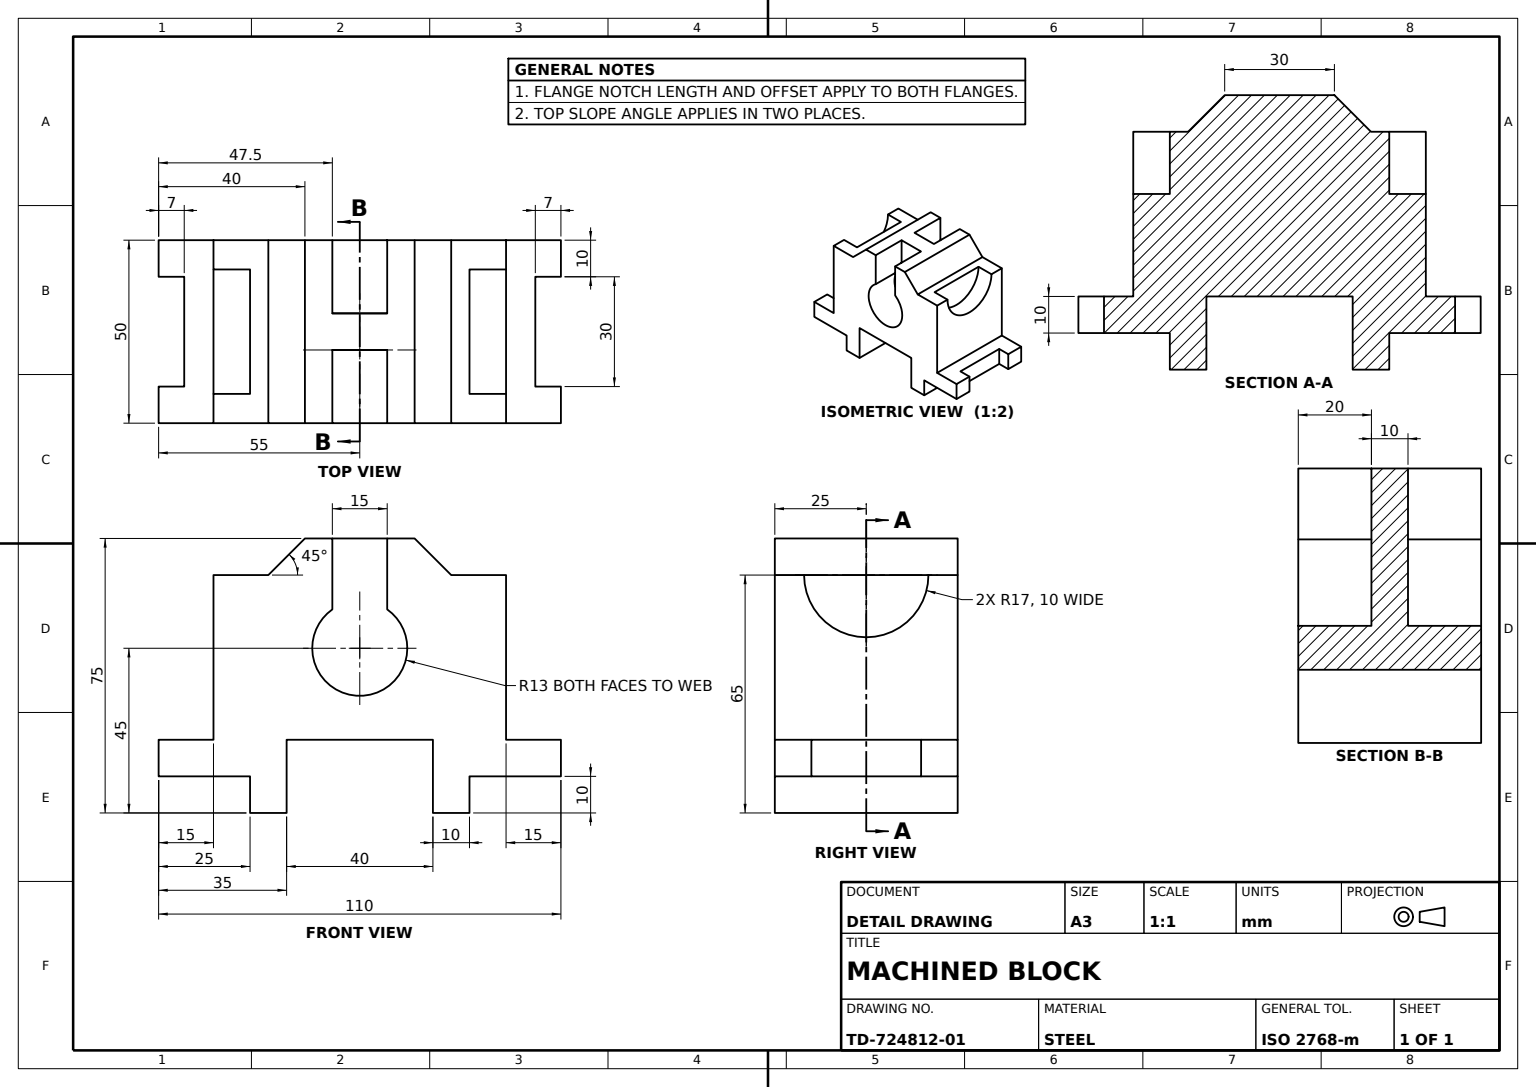
ISO-10303-21;
HEADER;
FILE_DESCRIPTION((''),'2;1');
FILE_NAME('','',(''),(''),'','','');
FILE_SCHEMA(('AUTOMOTIVE_DESIGN'));
ENDSEC;
DATA;
#1=APPLICATION_CONTEXT('');
#2=PRODUCT_CONTEXT('',#1,'mechanical');
#3=PRODUCT('','','',(#2));
#4=PRODUCT_DEFINITION_FORMATION('','',#3);
#5=PRODUCT_DEFINITION_CONTEXT('',#1,'design');
#6=PRODUCT_DEFINITION('','',#4,#5);
#7=PRODUCT_DEFINITION_SHAPE('','',#6);
#8=(LENGTH_UNIT()NAMED_UNIT(*)SI_UNIT(.MILLI.,.METRE.));
#9=(NAMED_UNIT(*)PLANE_ANGLE_UNIT()SI_UNIT($,.RADIAN.));
#10=(NAMED_UNIT(*)SI_UNIT($,.STERADIAN.)SOLID_ANGLE_UNIT());
#11=UNCERTAINTY_MEASURE_WITH_UNIT(LENGTH_MEASURE(1.E-05),#8,'distance_accuracy_value','');
#12=(GEOMETRIC_REPRESENTATION_CONTEXT(3)GLOBAL_UNCERTAINTY_ASSIGNED_CONTEXT((#11))GLOBAL_UNIT_ASSIGNED_CONTEXT((#8,#9,#10))REPRESENTATION_CONTEXT('',''));
#13=CARTESIAN_POINT('',(110.,10.,10.));
#14=VERTEX_POINT('',#13);
#15=CARTESIAN_POINT('',(110.,10.,0.));
#16=VERTEX_POINT('',#15);
#17=CARTESIAN_POINT('',(110.,10.,50.));
#18=DIRECTION('',(0.,0.,-1.));
#19=VECTOR('',#18,1000.);
#20=LINE('',#17,#19);
#21=EDGE_CURVE('',#14,#16,#20,.T.);
#22=ORIENTED_EDGE('',*,*,#21,.F.);
#23=CARTESIAN_POINT('',(110.,0.,10.));
#24=VERTEX_POINT('',#23);
#25=DIRECTION('',(0.,1.,0.));
#26=VECTOR('',#25,1000.);
#27=LINE('',#23,#26);
#28=EDGE_CURVE('',#24,#14,#27,.T.);
#29=ORIENTED_EDGE('',*,*,#28,.F.);
#30=CARTESIAN_POINT('',(110.,0.,0.));
#31=VERTEX_POINT('',#30);
#32=CARTESIAN_POINT('',(110.,0.,50.));
#33=LINE('',#32,#19);
#34=EDGE_CURVE('',#24,#31,#33,.T.);
#35=ORIENTED_EDGE('',*,*,#34,.T.);
#36=LINE('',#30,#26);
#37=EDGE_CURVE('',#31,#16,#36,.T.);
#38=ORIENTED_EDGE('',*,*,#37,.T.);
#39=EDGE_LOOP('',(#22,#29,#35,#38));
#40=FACE_OUTER_BOUND('',#39,.T.);
#41=DIRECTION('',(-1.,0.,0.));
#42=DIRECTION('',(0.,0.,1.));
#43=AXIS2_PLACEMENT_3D('',#32,#41,#42);
#44=PLANE('',#43);
#45=ADVANCED_FACE('',(#40),#44,.F.);
#46=CARTESIAN_POINT('',(47.5,65.,20.));
#47=VERTEX_POINT('',#46);
#48=CARTESIAN_POINT('',(47.5,65.,0.));
#49=VERTEX_POINT('',#48);
#50=CARTESIAN_POINT('',(47.5,65.,50.));
#51=LINE('',#50,#19);
#52=EDGE_CURVE('',#47,#49,#51,.T.);
#53=ORIENTED_EDGE('',*,*,#52,.F.);
#54=CARTESIAN_POINT('',(47.5,45.61838,20.));
#55=VERTEX_POINT('',#54);
#56=CARTESIAN_POINT('',(47.5,15.,20.));
#57=LINE('',#56,#26);
#58=EDGE_CURVE('',#55,#47,#57,.T.);
#59=ORIENTED_EDGE('',*,*,#58,.F.);
#60=CARTESIAN_POINT('',(47.5,45.61838,0.));
#61=VERTEX_POINT('',#60);
#62=CARTESIAN_POINT('',(47.5,45.61838,50.));
#63=LINE('',#62,#19);
#64=EDGE_CURVE('',#55,#61,#63,.T.);
#65=ORIENTED_EDGE('',*,*,#64,.T.);
#66=LINE('',#48,#26);
#67=EDGE_CURVE('',#61,#49,#66,.T.);
#68=ORIENTED_EDGE('',*,*,#67,.T.);
#69=EDGE_LOOP('',(#53,#59,#65,#68));
#70=FACE_OUTER_BOUND('',#69,.T.);
#71=AXIS2_PLACEMENT_3D('',#50,#41,#42);
#72=PLANE('',#71);
#73=ADVANCED_FACE('',(#70),#72,.F.);
#74=CARTESIAN_POINT('',(95.,55.,42.));
#75=VERTEX_POINT('',#74);
#76=CARTESIAN_POINT('',(95.,55.,8.));
#77=VERTEX_POINT('',#76);
#78=CARTESIAN_POINT('',(95.,55.,25.));
#79=DIRECTION('',(1.,0.,0.));
#80=AXIS2_PLACEMENT_3D('',#78,#79,#18);
#81=CIRCLE('',#80,17.);
#82=EDGE_CURVE('',#75,#77,#81,.T.);
#83=ORIENTED_EDGE('',*,*,#82,.T.);
#84=CARTESIAN_POINT('',(85.,55.,8.));
#85=VERTEX_POINT('',#84);
#86=VECTOR('',#79,1000.);
#87=LINE('',#84,#86);
#88=EDGE_CURVE('',#85,#77,#87,.T.);
#89=ORIENTED_EDGE('',*,*,#88,.F.);
#90=CARTESIAN_POINT('',(85.,55.,42.));
#91=VERTEX_POINT('',#90);
#92=CARTESIAN_POINT('',(85.,55.,25.));
#93=AXIS2_PLACEMENT_3D('',#92,#79,#18);
#94=CIRCLE('',#93,17.);
#95=EDGE_CURVE('',#91,#85,#94,.T.);
#96=ORIENTED_EDGE('',*,*,#95,.F.);
#97=LINE('',#90,#86);
#98=EDGE_CURVE('',#91,#75,#97,.T.);
#99=ORIENTED_EDGE('',*,*,#98,.T.);
#100=EDGE_LOOP('',(#83,#89,#96,#99));
#101=FACE_OUTER_BOUND('',#100,.T.);
#102=CYLINDRICAL_SURFACE('',#93,17.);
#103=ADVANCED_FACE('',(#101),#102,.F.);
#104=CARTESIAN_POINT('',(15.,55.,8.));
#105=VERTEX_POINT('',#104);
#106=CARTESIAN_POINT('',(15.,55.,42.));
#107=VERTEX_POINT('',#106);
#108=CARTESIAN_POINT('',(15.,55.,25.));
#109=AXIS2_PLACEMENT_3D('',#108,#41,#42);
#110=CIRCLE('',#109,17.);
#111=EDGE_CURVE('',#105,#107,#110,.T.);
#112=ORIENTED_EDGE('',*,*,#111,.T.);
#113=CARTESIAN_POINT('',(25.,55.,42.));
#114=VERTEX_POINT('',#113);
#115=VECTOR('',#41,1000.);
#116=LINE('',#113,#115);
#117=EDGE_CURVE('',#114,#107,#116,.T.);
#118=ORIENTED_EDGE('',*,*,#117,.F.);
#119=CARTESIAN_POINT('',(25.,55.,8.));
#120=VERTEX_POINT('',#119);
#121=CARTESIAN_POINT('',(25.,55.,25.));
#122=AXIS2_PLACEMENT_3D('',#121,#41,#42);
#123=CIRCLE('',#122,17.);
#124=EDGE_CURVE('',#120,#114,#123,.T.);
#125=ORIENTED_EDGE('',*,*,#124,.F.);
#126=LINE('',#119,#115);
#127=EDGE_CURVE('',#120,#105,#126,.T.);
#128=ORIENTED_EDGE('',*,*,#127,.T.);
#129=EDGE_LOOP('',(#112,#118,#125,#128));
#130=FACE_OUTER_BOUND('',#129,.T.);
#131=CYLINDRICAL_SURFACE('',#122,17.);
#132=ADVANCED_FACE('',(#130),#131,.F.);
#133=CARTESIAN_POINT('',(7.,0.,10.));
#134=VERTEX_POINT('',#133);
#135=CARTESIAN_POINT('',(0.,0.,10.));
#136=VERTEX_POINT('',#135);
#137=LINE('',#133,#115);
#138=EDGE_CURVE('',#134,#136,#137,.T.);
#139=ORIENTED_EDGE('',*,*,#138,.F.);
#140=CARTESIAN_POINT('',(7.,10.,10.));
#141=VERTEX_POINT('',#140);
#142=DIRECTION('',(0.,-1.,0.));
#143=VECTOR('',#142,1000.);
#144=LINE('',#140,#143);
#145=EDGE_CURVE('',#141,#134,#144,.T.);
#146=ORIENTED_EDGE('',*,*,#145,.F.);
#147=CARTESIAN_POINT('',(0.,10.,10.));
#148=VERTEX_POINT('',#147);
#149=LINE('',#140,#115);
#150=EDGE_CURVE('',#141,#148,#149,.T.);
#151=ORIENTED_EDGE('',*,*,#150,.T.);
#152=LINE('',#147,#143);
#153=EDGE_CURVE('',#148,#136,#152,.T.);
#154=ORIENTED_EDGE('',*,*,#153,.T.);
#155=EDGE_LOOP('',(#139,#146,#151,#154));
#156=FACE_OUTER_BOUND('',#155,.T.);
#157=AXIS2_PLACEMENT_3D('',#140,#18,#41);
#158=PLANE('',#157);
#159=ADVANCED_FACE('',(#156),#158,.F.);
#160=CARTESIAN_POINT('',(95.,10.,50.));
#161=VERTEX_POINT('',#160);
#162=CARTESIAN_POINT('',(95.,10.,0.));
#163=VERTEX_POINT('',#162);
#164=LINE('',#160,#19);
#165=EDGE_CURVE('',#161,#163,#164,.T.);
#166=ORIENTED_EDGE('',*,*,#165,.T.);
#167=CARTESIAN_POINT('',(95.,55.,0.));
#168=VERTEX_POINT('',#167);
#169=LINE('',#162,#26);
#170=EDGE_CURVE('',#163,#168,#169,.T.);
#171=ORIENTED_EDGE('',*,*,#170,.T.);
#172=CARTESIAN_POINT('',(95.,55.,50.));
#173=LINE('',#172,#19);
#174=EDGE_CURVE('',#77,#168,#173,.T.);
#175=ORIENTED_EDGE('',*,*,#174,.F.);
#176=ORIENTED_EDGE('',*,*,#82,.F.);
#177=VERTEX_POINT('',#172);
#178=EDGE_CURVE('',#177,#75,#173,.T.);
#179=ORIENTED_EDGE('',*,*,#178,.F.);
#180=LINE('',#160,#26);
#181=EDGE_CURVE('',#161,#177,#180,.T.);
#182=ORIENTED_EDGE('',*,*,#181,.F.);
#183=EDGE_LOOP('',(#166,#171,#175,#176,#179,#182));
#184=FACE_OUTER_BOUND('',#183,.T.);
#185=AXIS2_PLACEMENT_3D('',#160,#41,#42);
#186=PLANE('',#185);
#187=ADVANCED_FACE('',(#184),#186,.F.);
#188=CARTESIAN_POINT('',(35.,-10.,50.));
#189=VERTEX_POINT('',#188);
#190=CARTESIAN_POINT('',(35.,-10.,0.));
#191=VERTEX_POINT('',#190);
#192=LINE('',#188,#19);
#193=EDGE_CURVE('',#189,#191,#192,.T.);
#194=ORIENTED_EDGE('',*,*,#193,.F.);
#195=CARTESIAN_POINT('',(25.,-10.,50.));
#196=VERTEX_POINT('',#195);
#197=LINE('',#195,#86);
#198=EDGE_CURVE('',#196,#189,#197,.T.);
#199=ORIENTED_EDGE('',*,*,#198,.F.);
#200=CARTESIAN_POINT('',(25.,-10.,0.));
#201=VERTEX_POINT('',#200);
#202=LINE('',#195,#19);
#203=EDGE_CURVE('',#196,#201,#202,.T.);
#204=ORIENTED_EDGE('',*,*,#203,.T.);
#205=LINE('',#200,#86);
#206=EDGE_CURVE('',#201,#191,#205,.T.);
#207=ORIENTED_EDGE('',*,*,#206,.T.);
#208=EDGE_LOOP('',(#194,#199,#204,#207));
#209=FACE_OUTER_BOUND('',#208,.T.);
#210=AXIS2_PLACEMENT_3D('',#195,#25,#42);
#211=PLANE('',#210);
#212=ADVANCED_FACE('',(#209),#211,.F.);
#213=CARTESIAN_POINT('',(47.5,65.,30.));
#214=VERTEX_POINT('',#213);
#215=CARTESIAN_POINT('',(62.5,65.,30.));
#216=VERTEX_POINT('',#215);
#217=CARTESIAN_POINT('',(0.,65.,30.));
#218=LINE('',#217,#86);
#219=EDGE_CURVE('',#214,#216,#218,.T.);
#220=ORIENTED_EDGE('',*,*,#219,.F.);
#221=CARTESIAN_POINT('',(47.5,45.61838,30.));
#222=VERTEX_POINT('',#221);
#223=CARTESIAN_POINT('',(47.5,15.,30.));
#224=LINE('',#223,#26);
#225=EDGE_CURVE('',#222,#214,#224,.T.);
#226=ORIENTED_EDGE('',*,*,#225,.F.);
#227=CARTESIAN_POINT('',(42.,35.,30.));
#228=VERTEX_POINT('',#227);
#229=CARTESIAN_POINT('',(55.,35.,30.));
#230=AXIS2_PLACEMENT_3D('',#229,#18,#79);
#231=CIRCLE('',#230,13.);
#232=EDGE_CURVE('',#228,#222,#231,.T.);
#233=ORIENTED_EDGE('',*,*,#232,.F.);
#234=CARTESIAN_POINT('',(68.,35.,30.));
#235=VERTEX_POINT('',#234);
#236=EDGE_CURVE('',#235,#228,#231,.T.);
#237=ORIENTED_EDGE('',*,*,#236,.F.);
#238=CARTESIAN_POINT('',(62.5,45.61838,30.));
#239=VERTEX_POINT('',#238);
#240=EDGE_CURVE('',#239,#235,#231,.T.);
#241=ORIENTED_EDGE('',*,*,#240,.F.);
#242=CARTESIAN_POINT('',(62.5,15.,30.));
#243=LINE('',#242,#26);
#244=EDGE_CURVE('',#239,#216,#243,.T.);
#245=ORIENTED_EDGE('',*,*,#244,.T.);
#246=EDGE_LOOP('',(#220,#226,#233,#237,#241,#245));
#247=FACE_OUTER_BOUND('',#246,.T.);
#248=CARTESIAN_POINT('',(0.,15.,30.));
#249=AXIS2_PLACEMENT_3D('',#248,#42,#79);
#250=PLANE('',#249);
#251=ADVANCED_FACE('',(#247),#250,.T.);
#252=CARTESIAN_POINT('',(25.,0.,0.));
#253=VERTEX_POINT('',#252);
#254=LINE('',#252,#143);
#255=EDGE_CURVE('',#253,#201,#254,.T.);
#256=ORIENTED_EDGE('',*,*,#255,.T.);
#257=ORIENTED_EDGE('',*,*,#203,.F.);
#258=CARTESIAN_POINT('',(25.,0.,50.));
#259=VERTEX_POINT('',#258);
#260=LINE('',#258,#143);
#261=EDGE_CURVE('',#259,#196,#260,.T.);
#262=ORIENTED_EDGE('',*,*,#261,.F.);
#263=LINE('',#258,#19);
#264=EDGE_CURVE('',#259,#253,#263,.T.);
#265=ORIENTED_EDGE('',*,*,#264,.T.);
#266=EDGE_LOOP('',(#256,#257,#262,#265));
#267=FACE_OUTER_BOUND('',#266,.T.);
#268=AXIS2_PLACEMENT_3D('',#258,#79,#18);
#269=PLANE('',#268);
#270=ADVANCED_FACE('',(#267),#269,.F.);
#271=ORIENTED_EDGE('',*,*,#34,.F.);
#272=CARTESIAN_POINT('',(103.,0.,10.));
#273=VERTEX_POINT('',#272);
#274=LINE('',#272,#86);
#275=EDGE_CURVE('',#273,#24,#274,.T.);
#276=ORIENTED_EDGE('',*,*,#275,.F.);
#277=CARTESIAN_POINT('',(103.,0.,40.));
#278=VERTEX_POINT('',#277);
#279=LINE('',#277,#19);
#280=EDGE_CURVE('',#278,#273,#279,.T.);
#281=ORIENTED_EDGE('',*,*,#280,.F.);
#282=CARTESIAN_POINT('',(110.,0.,40.));
#283=VERTEX_POINT('',#282);
#284=LINE('',#277,#86);
#285=EDGE_CURVE('',#278,#283,#284,.T.);
#286=ORIENTED_EDGE('',*,*,#285,.T.);
#287=VERTEX_POINT('',#32);
#288=EDGE_CURVE('',#287,#283,#33,.T.);
#289=ORIENTED_EDGE('',*,*,#288,.F.);
#290=CARTESIAN_POINT('',(85.,0.,50.));
#291=VERTEX_POINT('',#290);
#292=LINE('',#290,#86);
#293=EDGE_CURVE('',#291,#287,#292,.T.);
#294=ORIENTED_EDGE('',*,*,#293,.F.);
#295=CARTESIAN_POINT('',(85.,0.,0.));
#296=VERTEX_POINT('',#295);
#297=LINE('',#290,#19);
#298=EDGE_CURVE('',#291,#296,#297,.T.);
#299=ORIENTED_EDGE('',*,*,#298,.T.);
#300=LINE('',#295,#86);
#301=EDGE_CURVE('',#296,#31,#300,.T.);
#302=ORIENTED_EDGE('',*,*,#301,.T.);
#303=EDGE_LOOP('',(#271,#276,#281,#286,#289,#294,#299,#302));
#304=FACE_OUTER_BOUND('',#303,.T.);
#305=AXIS2_PLACEMENT_3D('',#290,#25,#42);
#306=PLANE('',#305);
#307=ADVANCED_FACE('',(#304),#306,.F.);
#308=VERTEX_POINT('',#17);
#309=LINE('',#32,#26);
#310=EDGE_CURVE('',#287,#308,#309,.T.);
#311=ORIENTED_EDGE('',*,*,#310,.F.);
#312=ORIENTED_EDGE('',*,*,#288,.T.);
#313=CARTESIAN_POINT('',(110.,10.,40.));
#314=VERTEX_POINT('',#313);
#315=LINE('',#313,#143);
#316=EDGE_CURVE('',#314,#283,#315,.T.);
#317=ORIENTED_EDGE('',*,*,#316,.F.);
#318=EDGE_CURVE('',#308,#314,#20,.T.);
#319=ORIENTED_EDGE('',*,*,#318,.F.);
#320=EDGE_LOOP('',(#311,#312,#317,#319));
#321=FACE_OUTER_BOUND('',#320,.T.);
#322=ADVANCED_FACE('',(#321),#44,.F.);
#323=CARTESIAN_POINT('',(68.,35.,50.));
#324=VERTEX_POINT('',#323);
#325=CARTESIAN_POINT('',(42.,35.,50.));
#326=VERTEX_POINT('',#325);
#327=CARTESIAN_POINT('',(55.,35.,50.));
#328=AXIS2_PLACEMENT_3D('',#327,#18,#79);
#329=CIRCLE('',#328,13.);
#330=EDGE_CURVE('',#324,#326,#329,.T.);
#331=ORIENTED_EDGE('',*,*,#330,.F.);
#332=LINE('',#323,#19);
#333=EDGE_CURVE('',#324,#235,#332,.T.);
#334=ORIENTED_EDGE('',*,*,#333,.T.);
#335=ORIENTED_EDGE('',*,*,#236,.T.);
#336=LINE('',#325,#19);
#337=EDGE_CURVE('',#326,#228,#336,.T.);
#338=ORIENTED_EDGE('',*,*,#337,.F.);
#339=EDGE_LOOP('',(#331,#334,#335,#338));
#340=FACE_OUTER_BOUND('',#339,.T.);
#341=AXIS2_PLACEMENT_3D('',#327,#18,#41);
#342=CYLINDRICAL_SURFACE('',#341,13.);
#343=ADVANCED_FACE('',(#340),#342,.F.);
#344=CARTESIAN_POINT('',(15.,55.,50.));
#345=VERTEX_POINT('',#344);
#346=LINE('',#344,#19);
#347=EDGE_CURVE('',#345,#107,#346,.T.);
#348=ORIENTED_EDGE('',*,*,#347,.T.);
#349=ORIENTED_EDGE('',*,*,#111,.F.);
#350=CARTESIAN_POINT('',(15.,55.,0.));
#351=VERTEX_POINT('',#350);
#352=EDGE_CURVE('',#105,#351,#346,.T.);
#353=ORIENTED_EDGE('',*,*,#352,.T.);
#354=CARTESIAN_POINT('',(15.,10.,0.));
#355=VERTEX_POINT('',#354);
#356=LINE('',#354,#143);
#357=EDGE_CURVE('',#351,#355,#356,.T.);
#358=ORIENTED_EDGE('',*,*,#357,.T.);
#359=CARTESIAN_POINT('',(15.,10.,50.));
#360=VERTEX_POINT('',#359);
#361=LINE('',#359,#19);
#362=EDGE_CURVE('',#360,#355,#361,.T.);
#363=ORIENTED_EDGE('',*,*,#362,.F.);
#364=LINE('',#359,#143);
#365=EDGE_CURVE('',#345,#360,#364,.T.);
#366=ORIENTED_EDGE('',*,*,#365,.F.);
#367=EDGE_LOOP('',(#348,#349,#353,#358,#363,#366));
#368=FACE_OUTER_BOUND('',#367,.T.);
#369=AXIS2_PLACEMENT_3D('',#359,#79,#18);
#370=PLANE('',#369);
#371=ADVANCED_FACE('',(#368),#370,.F.);
#372=CARTESIAN_POINT('',(40.,65.,0.));
#373=VERTEX_POINT('',#372);
#374=CARTESIAN_POINT('',(30.,55.,0.));
#375=VERTEX_POINT('',#374);
#376=DIRECTION('',(-0.707106781,-0.707106781,0.));
#377=VECTOR('',#376,1000.);
#378=LINE('',#372,#377);
#379=EDGE_CURVE('',#373,#375,#378,.T.);
#380=ORIENTED_EDGE('',*,*,#379,.F.);
#381=LINE('',#48,#115);
#382=EDGE_CURVE('',#49,#373,#381,.T.);
#383=ORIENTED_EDGE('',*,*,#382,.F.);
#384=ORIENTED_EDGE('',*,*,#67,.F.);
#385=CARTESIAN_POINT('',(42.,35.,0.));
#386=VERTEX_POINT('',#385);
#387=CARTESIAN_POINT('',(55.,35.,0.));
#388=AXIS2_PLACEMENT_3D('',#387,#18,#79);
#389=CIRCLE('',#388,13.);
#390=EDGE_CURVE('',#386,#61,#389,.T.);
#391=ORIENTED_EDGE('',*,*,#390,.F.);
#392=CARTESIAN_POINT('',(68.,35.,0.));
#393=VERTEX_POINT('',#392);
#394=EDGE_CURVE('',#393,#386,#389,.T.);
#395=ORIENTED_EDGE('',*,*,#394,.F.);
#396=CARTESIAN_POINT('',(62.5,45.61838,0.));
#397=VERTEX_POINT('',#396);
#398=EDGE_CURVE('',#397,#393,#389,.T.);
#399=ORIENTED_EDGE('',*,*,#398,.F.);
#400=CARTESIAN_POINT('',(62.5,65.,0.));
#401=VERTEX_POINT('',#400);
#402=CARTESIAN_POINT('',(62.5,48.,0.));
#403=LINE('',#402,#143);
#404=EDGE_CURVE('',#401,#397,#403,.T.);
#405=ORIENTED_EDGE('',*,*,#404,.F.);
#406=CARTESIAN_POINT('',(70.,65.,0.));
#407=VERTEX_POINT('',#406);
#408=LINE('',#400,#115);
#409=EDGE_CURVE('',#407,#401,#408,.T.);
#410=ORIENTED_EDGE('',*,*,#409,.F.);
#411=CARTESIAN_POINT('',(80.,55.,0.));
#412=VERTEX_POINT('',#411);
#413=DIRECTION('',(-0.707106781,0.707106781,0.));
#414=VECTOR('',#413,1000.);
#415=LINE('',#406,#414);
#416=EDGE_CURVE('',#412,#407,#415,.T.);
#417=ORIENTED_EDGE('',*,*,#416,.F.);
#418=LINE('',#167,#115);
#419=EDGE_CURVE('',#168,#412,#418,.T.);
#420=ORIENTED_EDGE('',*,*,#419,.F.);
#421=ORIENTED_EDGE('',*,*,#170,.F.);
#422=LINE('',#15,#115);
#423=EDGE_CURVE('',#16,#163,#422,.T.);
#424=ORIENTED_EDGE('',*,*,#423,.F.);
#425=ORIENTED_EDGE('',*,*,#37,.F.);
#426=ORIENTED_EDGE('',*,*,#301,.F.);
#427=CARTESIAN_POINT('',(85.,-10.,0.));
#428=VERTEX_POINT('',#427);
#429=LINE('',#427,#26);
#430=EDGE_CURVE('',#428,#296,#429,.T.);
#431=ORIENTED_EDGE('',*,*,#430,.F.);
#432=CARTESIAN_POINT('',(75.,-10.,0.));
#433=VERTEX_POINT('',#432);
#434=LINE('',#432,#86);
#435=EDGE_CURVE('',#433,#428,#434,.T.);
#436=ORIENTED_EDGE('',*,*,#435,.F.);
#437=CARTESIAN_POINT('',(75.,10.,0.));
#438=VERTEX_POINT('',#437);
#439=LINE('',#437,#143);
#440=EDGE_CURVE('',#438,#433,#439,.T.);
#441=ORIENTED_EDGE('',*,*,#440,.F.);
#442=CARTESIAN_POINT('',(35.,10.,0.));
#443=VERTEX_POINT('',#442);
#444=LINE('',#442,#86);
#445=EDGE_CURVE('',#443,#438,#444,.T.);
#446=ORIENTED_EDGE('',*,*,#445,.F.);
#447=LINE('',#190,#26);
#448=EDGE_CURVE('',#191,#443,#447,.T.);
#449=ORIENTED_EDGE('',*,*,#448,.F.);
#450=ORIENTED_EDGE('',*,*,#206,.F.);
#451=ORIENTED_EDGE('',*,*,#255,.F.);
#452=CARTESIAN_POINT('',(0.,0.,0.));
#453=VERTEX_POINT('',#452);
#454=LINE('',#452,#86);
#455=EDGE_CURVE('',#453,#253,#454,.T.);
#456=ORIENTED_EDGE('',*,*,#455,.F.);
#457=CARTESIAN_POINT('',(0.,10.,0.));
#458=VERTEX_POINT('',#457);
#459=LINE('',#457,#143);
#460=EDGE_CURVE('',#458,#453,#459,.T.);
#461=ORIENTED_EDGE('',*,*,#460,.F.);
#462=LINE('',#354,#115);
#463=EDGE_CURVE('',#355,#458,#462,.T.);
#464=ORIENTED_EDGE('',*,*,#463,.F.);
#465=ORIENTED_EDGE('',*,*,#357,.F.);
#466=LINE('',#350,#115);
#467=EDGE_CURVE('',#375,#351,#466,.T.);
#468=ORIENTED_EDGE('',*,*,#467,.F.);
#469=EDGE_LOOP('',(#380,#383,#384,#391,#395,#399,#405,#410,#417,#420,#421,#424,#425,#426,#431,#436,#441,#446,#449,#450,#451,#456,#461,#464,#465,#468));
#470=FACE_OUTER_BOUND('',#469,.T.);
#471=AXIS2_PLACEMENT_3D('',#387,#42,#79);
#472=PLANE('',#471);
#473=ADVANCED_FACE('',(#470),#472,.F.);
#474=CARTESIAN_POINT('',(42.,35.,20.));
#475=VERTEX_POINT('',#474);
#476=CARTESIAN_POINT('',(68.,35.,20.));
#477=VERTEX_POINT('',#476);
#478=CARTESIAN_POINT('',(55.,35.,20.));
#479=AXIS2_PLACEMENT_3D('',#478,#42,#41);
#480=CIRCLE('',#479,13.);
#481=EDGE_CURVE('',#475,#477,#480,.T.);
#482=ORIENTED_EDGE('',*,*,#481,.T.);
#483=EDGE_CURVE('',#477,#393,#332,.T.);
#484=ORIENTED_EDGE('',*,*,#483,.T.);
#485=ORIENTED_EDGE('',*,*,#394,.T.);
#486=EDGE_CURVE('',#475,#386,#336,.T.);
#487=ORIENTED_EDGE('',*,*,#486,.F.);
#488=EDGE_LOOP('',(#482,#484,#485,#487));
#489=FACE_OUTER_BOUND('',#488,.T.);
#490=ADVANCED_FACE('',(#489),#342,.F.);
#491=CARTESIAN_POINT('',(30.,55.,50.));
#492=VERTEX_POINT('',#491);
#493=LINE('',#491,#19);
#494=EDGE_CURVE('',#492,#375,#493,.T.);
#495=ORIENTED_EDGE('',*,*,#494,.F.);
#496=CARTESIAN_POINT('',(40.,65.,50.));
#497=VERTEX_POINT('',#496);
#498=LINE('',#496,#377);
#499=EDGE_CURVE('',#497,#492,#498,.T.);
#500=ORIENTED_EDGE('',*,*,#499,.F.);
#501=LINE('',#496,#19);
#502=EDGE_CURVE('',#497,#373,#501,.T.);
#503=ORIENTED_EDGE('',*,*,#502,.T.);
#504=ORIENTED_EDGE('',*,*,#379,.T.);
#505=EDGE_LOOP('',(#495,#500,#503,#504));
#506=FACE_OUTER_BOUND('',#505,.T.);
#507=DIRECTION('',(0.707106781,-0.707106781,0.));
#508=DIRECTION('',(0.707106781,0.707106781,0.));
#509=AXIS2_PLACEMENT_3D('',#496,#507,#508);
#510=PLANE('',#509);
#511=ADVANCED_FACE('',(#506),#510,.F.);
#512=CARTESIAN_POINT('',(35.,10.,50.));
#513=VERTEX_POINT('',#512);
#514=LINE('',#188,#26);
#515=EDGE_CURVE('',#189,#513,#514,.T.);
#516=ORIENTED_EDGE('',*,*,#515,.F.);
#517=ORIENTED_EDGE('',*,*,#193,.T.);
#518=ORIENTED_EDGE('',*,*,#448,.T.);
#519=LINE('',#512,#19);
#520=EDGE_CURVE('',#513,#443,#519,.T.);
#521=ORIENTED_EDGE('',*,*,#520,.F.);
#522=EDGE_LOOP('',(#516,#517,#518,#521));
#523=FACE_OUTER_BOUND('',#522,.T.);
#524=AXIS2_PLACEMENT_3D('',#188,#41,#42);
#525=PLANE('',#524);
#526=ADVANCED_FACE('',(#523),#525,.F.);
#527=CARTESIAN_POINT('',(0.,10.,50.));
#528=VERTEX_POINT('',#527);
#529=LINE('',#359,#115);
#530=EDGE_CURVE('',#360,#528,#529,.T.);
#531=ORIENTED_EDGE('',*,*,#530,.F.);
#532=ORIENTED_EDGE('',*,*,#362,.T.);
#533=ORIENTED_EDGE('',*,*,#463,.T.);
#534=LINE('',#527,#19);
#535=EDGE_CURVE('',#148,#458,#534,.T.);
#536=ORIENTED_EDGE('',*,*,#535,.F.);
#537=ORIENTED_EDGE('',*,*,#150,.F.);
#538=CARTESIAN_POINT('',(7.,10.,40.));
#539=VERTEX_POINT('',#538);
#540=LINE('',#538,#19);
#541=EDGE_CURVE('',#539,#141,#540,.T.);
#542=ORIENTED_EDGE('',*,*,#541,.F.);
#543=CARTESIAN_POINT('',(0.,10.,40.));
#544=VERTEX_POINT('',#543);
#545=LINE('',#538,#115);
#546=EDGE_CURVE('',#539,#544,#545,.T.);
#547=ORIENTED_EDGE('',*,*,#546,.T.);
#548=EDGE_CURVE('',#528,#544,#534,.T.);
#549=ORIENTED_EDGE('',*,*,#548,.F.);
#550=EDGE_LOOP('',(#531,#532,#533,#536,#537,#542,#547,#549));
#551=FACE_OUTER_BOUND('',#550,.T.);
#552=AXIS2_PLACEMENT_3D('',#359,#142,#18);
#553=PLANE('',#552);
#554=ADVANCED_FACE('',(#551),#553,.F.);
#555=ORIENTED_EDGE('',*,*,#352,.F.);
#556=ORIENTED_EDGE('',*,*,#127,.F.);
#557=LINE('',#119,#19);
#558=EDGE_CURVE('',#114,#120,#557,.T.);
#559=ORIENTED_EDGE('',*,*,#558,.F.);
#560=ORIENTED_EDGE('',*,*,#117,.T.);
#561=ORIENTED_EDGE('',*,*,#347,.F.);
#562=LINE('',#344,#115);
#563=EDGE_CURVE('',#492,#345,#562,.T.);
#564=ORIENTED_EDGE('',*,*,#563,.F.);
#565=ORIENTED_EDGE('',*,*,#494,.T.);
#566=ORIENTED_EDGE('',*,*,#467,.T.);
#567=EDGE_LOOP('',(#555,#556,#559,#560,#561,#564,#565,#566));
#568=FACE_OUTER_BOUND('',#567,.T.);
#569=AXIS2_PLACEMENT_3D('',#344,#142,#18);
#570=PLANE('',#569);
#571=ADVANCED_FACE('',(#568),#570,.F.);
#572=ORIENTED_EDGE('',*,*,#244,.F.);
#573=CARTESIAN_POINT('',(62.5,45.61838,50.));
#574=VERTEX_POINT('',#573);
#575=LINE('',#573,#19);
#576=EDGE_CURVE('',#574,#239,#575,.T.);
#577=ORIENTED_EDGE('',*,*,#576,.F.);
#578=CARTESIAN_POINT('',(62.5,65.,50.));
#579=VERTEX_POINT('',#578);
#580=CARTESIAN_POINT('',(62.5,48.,50.));
#581=LINE('',#580,#143);
#582=EDGE_CURVE('',#579,#574,#581,.T.);
#583=ORIENTED_EDGE('',*,*,#582,.F.);
#584=LINE('',#578,#19);
#585=EDGE_CURVE('',#579,#216,#584,.T.);
#586=ORIENTED_EDGE('',*,*,#585,.T.);
#587=EDGE_LOOP('',(#572,#577,#583,#586));
#588=FACE_OUTER_BOUND('',#587,.T.);
#589=AXIS2_PLACEMENT_3D('',#580,#79,#18);
#590=PLANE('',#589);
#591=ADVANCED_FACE('',(#588),#590,.F.);
#592=ORIENTED_EDGE('',*,*,#481,.F.);
#593=EDGE_CURVE('',#55,#475,#480,.T.);
#594=ORIENTED_EDGE('',*,*,#593,.F.);
#595=ORIENTED_EDGE('',*,*,#58,.T.);
#596=CARTESIAN_POINT('',(62.5,65.,20.));
#597=VERTEX_POINT('',#596);
#598=CARTESIAN_POINT('',(0.,65.,20.));
#599=LINE('',#598,#115);
#600=EDGE_CURVE('',#597,#47,#599,.T.);
#601=ORIENTED_EDGE('',*,*,#600,.F.);
#602=CARTESIAN_POINT('',(62.5,45.61838,20.));
#603=VERTEX_POINT('',#602);
#604=CARTESIAN_POINT('',(62.5,15.,20.));
#605=LINE('',#604,#26);
#606=EDGE_CURVE('',#603,#597,#605,.T.);
#607=ORIENTED_EDGE('',*,*,#606,.F.);
#608=EDGE_CURVE('',#477,#603,#480,.T.);
#609=ORIENTED_EDGE('',*,*,#608,.F.);
#610=EDGE_LOOP('',(#592,#594,#595,#601,#607,#609));
#611=FACE_OUTER_BOUND('',#610,.T.);
#612=CARTESIAN_POINT('',(0.,15.,20.));
#613=AXIS2_PLACEMENT_3D('',#612,#18,#41);
#614=PLANE('',#613);
#615=ADVANCED_FACE('',(#611),#614,.T.);
#616=CARTESIAN_POINT('',(103.,10.,10.));
#617=VERTEX_POINT('',#616);
#618=CARTESIAN_POINT('',(103.,10.,40.));
#619=VERTEX_POINT('',#618);
#620=VECTOR('',#42,1000.);
#621=LINE('',#616,#620);
#622=EDGE_CURVE('',#617,#619,#621,.T.);
#623=ORIENTED_EDGE('',*,*,#622,.T.);
#624=LINE('',#618,#143);
#625=EDGE_CURVE('',#619,#278,#624,.T.);
#626=ORIENTED_EDGE('',*,*,#625,.T.);
#627=ORIENTED_EDGE('',*,*,#280,.T.);
#628=LINE('',#272,#26);
#629=EDGE_CURVE('',#273,#617,#628,.T.);
#630=ORIENTED_EDGE('',*,*,#629,.T.);
#631=EDGE_LOOP('',(#623,#626,#627,#630));
#632=FACE_OUTER_BOUND('',#631,.T.);
#633=CARTESIAN_POINT('',(103.,0.,0.));
#634=AXIS2_PLACEMENT_3D('',#633,#79,#18);
#635=PLANE('',#634);
#636=ADVANCED_FACE('',(#632),#635,.T.);
#637=EDGE_CURVE('',#597,#401,#584,.T.);
#638=ORIENTED_EDGE('',*,*,#637,.T.);
#639=ORIENTED_EDGE('',*,*,#404,.T.);
#640=EDGE_CURVE('',#603,#397,#575,.T.);
#641=ORIENTED_EDGE('',*,*,#640,.F.);
#642=ORIENTED_EDGE('',*,*,#606,.T.);
#643=EDGE_LOOP('',(#638,#639,#641,#642));
#644=FACE_OUTER_BOUND('',#643,.T.);
#645=ADVANCED_FACE('',(#644),#590,.F.);
#646=ORIENTED_EDGE('',*,*,#153,.F.);
#647=ORIENTED_EDGE('',*,*,#535,.T.);
#648=ORIENTED_EDGE('',*,*,#460,.T.);
#649=CARTESIAN_POINT('',(0.,0.,50.));
#650=LINE('',#649,#19);
#651=EDGE_CURVE('',#136,#453,#650,.T.);
#652=ORIENTED_EDGE('',*,*,#651,.F.);
#653=EDGE_LOOP('',(#646,#647,#648,#652));
#654=FACE_OUTER_BOUND('',#653,.T.);
#655=AXIS2_PLACEMENT_3D('',#527,#79,#18);
#656=PLANE('',#655);
#657=ADVANCED_FACE('',(#654),#656,.F.);
#658=CARTESIAN_POINT('',(80.,55.,50.));
#659=VERTEX_POINT('',#658);
#660=LINE('',#658,#19);
#661=EDGE_CURVE('',#659,#412,#660,.T.);
#662=ORIENTED_EDGE('',*,*,#661,.T.);
#663=ORIENTED_EDGE('',*,*,#416,.T.);
#664=CARTESIAN_POINT('',(70.,65.,50.));
#665=VERTEX_POINT('',#664);
#666=LINE('',#664,#19);
#667=EDGE_CURVE('',#665,#407,#666,.T.);
#668=ORIENTED_EDGE('',*,*,#667,.F.);
#669=LINE('',#664,#414);
#670=EDGE_CURVE('',#659,#665,#669,.T.);
#671=ORIENTED_EDGE('',*,*,#670,.F.);
#672=EDGE_LOOP('',(#662,#663,#668,#671));
#673=FACE_OUTER_BOUND('',#672,.T.);
#674=AXIS2_PLACEMENT_3D('',#664,#376,#507);
#675=PLANE('',#674);
#676=ADVANCED_FACE('',(#673),#675,.F.);
#677=ORIENTED_EDGE('',*,*,#285,.F.);
#678=ORIENTED_EDGE('',*,*,#625,.F.);
#679=LINE('',#618,#86);
#680=EDGE_CURVE('',#619,#314,#679,.T.);
#681=ORIENTED_EDGE('',*,*,#680,.T.);
#682=ORIENTED_EDGE('',*,*,#316,.T.);
#683=EDGE_LOOP('',(#677,#678,#681,#682));
#684=FACE_OUTER_BOUND('',#683,.T.);
#685=AXIS2_PLACEMENT_3D('',#618,#42,#79);
#686=PLANE('',#685);
#687=ADVANCED_FACE('',(#684),#686,.F.);
#688=ORIENTED_EDGE('',*,*,#298,.F.);
#689=CARTESIAN_POINT('',(85.,-10.,50.));
#690=VERTEX_POINT('',#689);
#691=LINE('',#689,#26);
#692=EDGE_CURVE('',#690,#291,#691,.T.);
#693=ORIENTED_EDGE('',*,*,#692,.F.);
#694=LINE('',#689,#19);
#695=EDGE_CURVE('',#690,#428,#694,.T.);
#696=ORIENTED_EDGE('',*,*,#695,.T.);
#697=ORIENTED_EDGE('',*,*,#430,.T.);
#698=EDGE_LOOP('',(#688,#693,#696,#697));
#699=FACE_OUTER_BOUND('',#698,.T.);
#700=AXIS2_PLACEMENT_3D('',#689,#41,#42);
#701=PLANE('',#700);
#702=ADVANCED_FACE('',(#699),#701,.F.);
#703=ORIENTED_EDGE('',*,*,#165,.F.);
#704=LINE('',#17,#115);
#705=EDGE_CURVE('',#308,#161,#704,.T.);
#706=ORIENTED_EDGE('',*,*,#705,.F.);
#707=ORIENTED_EDGE('',*,*,#318,.T.);
#708=ORIENTED_EDGE('',*,*,#680,.F.);
#709=ORIENTED_EDGE('',*,*,#622,.F.);
#710=LINE('',#616,#86);
#711=EDGE_CURVE('',#617,#14,#710,.T.);
#712=ORIENTED_EDGE('',*,*,#711,.T.);
#713=ORIENTED_EDGE('',*,*,#21,.T.);
#714=ORIENTED_EDGE('',*,*,#423,.T.);
#715=EDGE_LOOP('',(#703,#706,#707,#708,#709,#712,#713,#714));
#716=FACE_OUTER_BOUND('',#715,.T.);
#717=AXIS2_PLACEMENT_3D('',#17,#142,#18);
#718=PLANE('',#717);
#719=ADVANCED_FACE('',(#716),#718,.F.);
#720=ORIENTED_EDGE('',*,*,#124,.T.);
#721=ORIENTED_EDGE('',*,*,#558,.T.);
#722=EDGE_LOOP('',(#720,#721));
#723=FACE_OUTER_BOUND('',#722,.T.);
#724=PLANE('',#122);
#725=ADVANCED_FACE('',(#723),#724,.T.);
#726=ORIENTED_EDGE('',*,*,#695,.F.);
#727=CARTESIAN_POINT('',(75.,-10.,50.));
#728=VERTEX_POINT('',#727);
#729=LINE('',#727,#86);
#730=EDGE_CURVE('',#728,#690,#729,.T.);
#731=ORIENTED_EDGE('',*,*,#730,.F.);
#732=LINE('',#727,#19);
#733=EDGE_CURVE('',#728,#433,#732,.T.);
#734=ORIENTED_EDGE('',*,*,#733,.T.);
#735=ORIENTED_EDGE('',*,*,#435,.T.);
#736=EDGE_LOOP('',(#726,#731,#734,#735));
#737=FACE_OUTER_BOUND('',#736,.T.);
#738=AXIS2_PLACEMENT_3D('',#727,#25,#42);
#739=PLANE('',#738);
#740=ADVANCED_FACE('',(#737),#739,.F.);
#741=VERTEX_POINT('',#649);
#742=CARTESIAN_POINT('',(0.,0.,40.));
#743=VERTEX_POINT('',#742);
#744=EDGE_CURVE('',#741,#743,#650,.T.);
#745=ORIENTED_EDGE('',*,*,#744,.T.);
#746=CARTESIAN_POINT('',(7.,0.,40.));
#747=VERTEX_POINT('',#746);
#748=LINE('',#746,#115);
#749=EDGE_CURVE('',#747,#743,#748,.T.);
#750=ORIENTED_EDGE('',*,*,#749,.F.);
#751=LINE('',#133,#620);
#752=EDGE_CURVE('',#134,#747,#751,.T.);
#753=ORIENTED_EDGE('',*,*,#752,.F.);
#754=ORIENTED_EDGE('',*,*,#138,.T.);
#755=ORIENTED_EDGE('',*,*,#651,.T.);
#756=ORIENTED_EDGE('',*,*,#455,.T.);
#757=ORIENTED_EDGE('',*,*,#264,.F.);
#758=LINE('',#649,#86);
#759=EDGE_CURVE('',#741,#259,#758,.T.);
#760=ORIENTED_EDGE('',*,*,#759,.F.);
#761=EDGE_LOOP('',(#745,#750,#753,#754,#755,#756,#757,#760));
#762=FACE_OUTER_BOUND('',#761,.T.);
#763=AXIS2_PLACEMENT_3D('',#649,#25,#42);
#764=PLANE('',#763);
#765=ADVANCED_FACE('',(#762),#764,.F.);
#766=ORIENTED_EDGE('',*,*,#733,.F.);
#767=CARTESIAN_POINT('',(75.,10.,50.));
#768=VERTEX_POINT('',#767);
#769=LINE('',#767,#143);
#770=EDGE_CURVE('',#768,#728,#769,.T.);
#771=ORIENTED_EDGE('',*,*,#770,.F.);
#772=LINE('',#767,#19);
#773=EDGE_CURVE('',#768,#438,#772,.T.);
#774=ORIENTED_EDGE('',*,*,#773,.T.);
#775=ORIENTED_EDGE('',*,*,#440,.T.);
#776=EDGE_LOOP('',(#766,#771,#774,#775));
#777=FACE_OUTER_BOUND('',#776,.T.);
#778=AXIS2_PLACEMENT_3D('',#767,#79,#18);
#779=PLANE('',#778);
#780=ADVANCED_FACE('',(#777),#779,.F.);
#781=VERTEX_POINT('',#62);
#782=EDGE_CURVE('',#781,#222,#63,.T.);
#783=ORIENTED_EDGE('',*,*,#782,.T.);
#784=ORIENTED_EDGE('',*,*,#225,.T.);
#785=VERTEX_POINT('',#50);
#786=EDGE_CURVE('',#785,#214,#51,.T.);
#787=ORIENTED_EDGE('',*,*,#786,.F.);
#788=CARTESIAN_POINT('',(47.5,48.,50.));
#789=LINE('',#788,#26);
#790=EDGE_CURVE('',#781,#785,#789,.T.);
#791=ORIENTED_EDGE('',*,*,#790,.F.);
#792=EDGE_LOOP('',(#783,#784,#787,#791));
#793=FACE_OUTER_BOUND('',#792,.T.);
#794=ADVANCED_FACE('',(#793),#72,.F.);
#795=ORIENTED_EDGE('',*,*,#790,.T.);
#796=LINE('',#50,#115);
#797=EDGE_CURVE('',#785,#497,#796,.T.);
#798=ORIENTED_EDGE('',*,*,#797,.T.);
#799=ORIENTED_EDGE('',*,*,#499,.T.);
#800=ORIENTED_EDGE('',*,*,#563,.T.);
#801=ORIENTED_EDGE('',*,*,#365,.T.);
#802=ORIENTED_EDGE('',*,*,#530,.T.);
#803=LINE('',#527,#143);
#804=EDGE_CURVE('',#528,#741,#803,.T.);
#805=ORIENTED_EDGE('',*,*,#804,.T.);
#806=ORIENTED_EDGE('',*,*,#759,.T.);
#807=ORIENTED_EDGE('',*,*,#261,.T.);
#808=ORIENTED_EDGE('',*,*,#198,.T.);
#809=ORIENTED_EDGE('',*,*,#515,.T.);
#810=LINE('',#512,#86);
#811=EDGE_CURVE('',#513,#768,#810,.T.);
#812=ORIENTED_EDGE('',*,*,#811,.T.);
#813=ORIENTED_EDGE('',*,*,#770,.T.);
#814=ORIENTED_EDGE('',*,*,#730,.T.);
#815=ORIENTED_EDGE('',*,*,#692,.T.);
#816=ORIENTED_EDGE('',*,*,#293,.T.);
#817=ORIENTED_EDGE('',*,*,#310,.T.);
#818=ORIENTED_EDGE('',*,*,#705,.T.);
#819=ORIENTED_EDGE('',*,*,#181,.T.);
#820=LINE('',#172,#115);
#821=EDGE_CURVE('',#177,#659,#820,.T.);
#822=ORIENTED_EDGE('',*,*,#821,.T.);
#823=ORIENTED_EDGE('',*,*,#670,.T.);
#824=LINE('',#578,#115);
#825=EDGE_CURVE('',#665,#579,#824,.T.);
#826=ORIENTED_EDGE('',*,*,#825,.T.);
#827=ORIENTED_EDGE('',*,*,#582,.T.);
#828=EDGE_CURVE('',#574,#324,#329,.T.);
#829=ORIENTED_EDGE('',*,*,#828,.T.);
#830=ORIENTED_EDGE('',*,*,#330,.T.);
#831=EDGE_CURVE('',#326,#781,#329,.T.);
#832=ORIENTED_EDGE('',*,*,#831,.T.);
#833=EDGE_LOOP('',(#795,#798,#799,#800,#801,#802,#805,#806,#807,#808,#809,#812,#813,#814,#815,#816,#817,#818,#819,#822,#823,#826,#827,#829,#830,#832));
#834=FACE_OUTER_BOUND('',#833,.T.);
#835=AXIS2_PLACEMENT_3D('',#327,#42,#79);
#836=PLANE('',#835);
#837=ADVANCED_FACE('',(#834),#836,.T.);
#838=ORIENTED_EDGE('',*,*,#831,.F.);
#839=ORIENTED_EDGE('',*,*,#337,.T.);
#840=ORIENTED_EDGE('',*,*,#232,.T.);
#841=ORIENTED_EDGE('',*,*,#782,.F.);
#842=EDGE_LOOP('',(#838,#839,#840,#841));
#843=FACE_OUTER_BOUND('',#842,.T.);
#844=ADVANCED_FACE('',(#843),#342,.F.);
#845=ORIENTED_EDGE('',*,*,#661,.F.);
#846=ORIENTED_EDGE('',*,*,#821,.F.);
#847=ORIENTED_EDGE('',*,*,#178,.T.);
#848=ORIENTED_EDGE('',*,*,#98,.F.);
#849=LINE('',#90,#620);
#850=EDGE_CURVE('',#85,#91,#849,.T.);
#851=ORIENTED_EDGE('',*,*,#850,.F.);
#852=ORIENTED_EDGE('',*,*,#88,.T.);
#853=ORIENTED_EDGE('',*,*,#174,.T.);
#854=ORIENTED_EDGE('',*,*,#419,.T.);
#855=EDGE_LOOP('',(#845,#846,#847,#848,#851,#852,#853,#854));
#856=FACE_OUTER_BOUND('',#855,.T.);
#857=AXIS2_PLACEMENT_3D('',#172,#142,#18);
#858=PLANE('',#857);
#859=ADVANCED_FACE('',(#856),#858,.F.);
#860=ORIENTED_EDGE('',*,*,#828,.F.);
#861=ORIENTED_EDGE('',*,*,#576,.T.);
#862=ORIENTED_EDGE('',*,*,#240,.T.);
#863=ORIENTED_EDGE('',*,*,#333,.F.);
#864=EDGE_LOOP('',(#860,#861,#862,#863));
#865=FACE_OUTER_BOUND('',#864,.T.);
#866=ADVANCED_FACE('',(#865),#342,.F.);
#867=ORIENTED_EDGE('',*,*,#786,.T.);
#868=ORIENTED_EDGE('',*,*,#219,.T.);
#869=ORIENTED_EDGE('',*,*,#585,.F.);
#870=ORIENTED_EDGE('',*,*,#825,.F.);
#871=ORIENTED_EDGE('',*,*,#667,.T.);
#872=ORIENTED_EDGE('',*,*,#409,.T.);
#873=ORIENTED_EDGE('',*,*,#637,.F.);
#874=ORIENTED_EDGE('',*,*,#600,.T.);
#875=ORIENTED_EDGE('',*,*,#52,.T.);
#876=ORIENTED_EDGE('',*,*,#382,.T.);
#877=ORIENTED_EDGE('',*,*,#502,.F.);
#878=ORIENTED_EDGE('',*,*,#797,.F.);
#879=EDGE_LOOP('',(#867,#868,#869,#870,#871,#872,#873,#874,#875,#876,#877,#878));
#880=FACE_OUTER_BOUND('',#879,.T.);
#881=AXIS2_PLACEMENT_3D('',#50,#142,#18);
#882=PLANE('',#881);
#883=ADVANCED_FACE('',(#880),#882,.F.);
#884=ORIENTED_EDGE('',*,*,#95,.T.);
#885=ORIENTED_EDGE('',*,*,#850,.T.);
#886=EDGE_LOOP('',(#884,#885));
#887=FACE_OUTER_BOUND('',#886,.T.);
#888=PLANE('',#93);
#889=ADVANCED_FACE('',(#887),#888,.T.);
#890=ORIENTED_EDGE('',*,*,#640,.T.);
#891=ORIENTED_EDGE('',*,*,#398,.T.);
#892=ORIENTED_EDGE('',*,*,#483,.F.);
#893=ORIENTED_EDGE('',*,*,#608,.T.);
#894=EDGE_LOOP('',(#890,#891,#892,#893));
#895=FACE_OUTER_BOUND('',#894,.T.);
#896=ADVANCED_FACE('',(#895),#342,.F.);
#897=ORIENTED_EDGE('',*,*,#546,.F.);
#898=LINE('',#746,#26);
#899=EDGE_CURVE('',#747,#539,#898,.T.);
#900=ORIENTED_EDGE('',*,*,#899,.F.);
#901=ORIENTED_EDGE('',*,*,#749,.T.);
#902=LINE('',#742,#26);
#903=EDGE_CURVE('',#743,#544,#902,.T.);
#904=ORIENTED_EDGE('',*,*,#903,.T.);
#905=EDGE_LOOP('',(#897,#900,#901,#904));
#906=FACE_OUTER_BOUND('',#905,.T.);
#907=AXIS2_PLACEMENT_3D('',#746,#42,#79);
#908=PLANE('',#907);
#909=ADVANCED_FACE('',(#906),#908,.F.);
#910=ORIENTED_EDGE('',*,*,#541,.T.);
#911=ORIENTED_EDGE('',*,*,#145,.T.);
#912=ORIENTED_EDGE('',*,*,#752,.T.);
#913=ORIENTED_EDGE('',*,*,#899,.T.);
#914=EDGE_LOOP('',(#910,#911,#912,#913));
#915=FACE_OUTER_BOUND('',#914,.T.);
#916=CARTESIAN_POINT('',(7.,0.,0.));
#917=AXIS2_PLACEMENT_3D('',#916,#41,#42);
#918=PLANE('',#917);
#919=ADVANCED_FACE('',(#915),#918,.T.);
#920=ORIENTED_EDGE('',*,*,#711,.F.);
#921=ORIENTED_EDGE('',*,*,#629,.F.);
#922=ORIENTED_EDGE('',*,*,#275,.T.);
#923=ORIENTED_EDGE('',*,*,#28,.T.);
#924=EDGE_LOOP('',(#920,#921,#922,#923));
#925=FACE_OUTER_BOUND('',#924,.T.);
#926=AXIS2_PLACEMENT_3D('',#272,#18,#41);
#927=PLANE('',#926);
#928=ADVANCED_FACE('',(#925),#927,.F.);
#929=ORIENTED_EDGE('',*,*,#486,.T.);
#930=ORIENTED_EDGE('',*,*,#390,.T.);
#931=ORIENTED_EDGE('',*,*,#64,.F.);
#932=ORIENTED_EDGE('',*,*,#593,.T.);
#933=EDGE_LOOP('',(#929,#930,#931,#932));
#934=FACE_OUTER_BOUND('',#933,.T.);
#935=ADVANCED_FACE('',(#934),#342,.F.);
#936=ORIENTED_EDGE('',*,*,#520,.T.);
#937=ORIENTED_EDGE('',*,*,#445,.T.);
#938=ORIENTED_EDGE('',*,*,#773,.F.);
#939=ORIENTED_EDGE('',*,*,#811,.F.);
#940=EDGE_LOOP('',(#936,#937,#938,#939));
#941=FACE_OUTER_BOUND('',#940,.T.);
#942=AXIS2_PLACEMENT_3D('',#512,#25,#42);
#943=PLANE('',#942);
#944=ADVANCED_FACE('',(#941),#943,.F.);
#945=ORIENTED_EDGE('',*,*,#804,.F.);
#946=ORIENTED_EDGE('',*,*,#548,.T.);
#947=ORIENTED_EDGE('',*,*,#903,.F.);
#948=ORIENTED_EDGE('',*,*,#744,.F.);
#949=EDGE_LOOP('',(#945,#946,#947,#948));
#950=FACE_OUTER_BOUND('',#949,.T.);
#951=ADVANCED_FACE('',(#950),#656,.F.);
#952=CLOSED_SHELL('',(#45,#73,#103,#132,#159,#187,#212,#251,#270,#307,#322,#343,#371,#473,#490,#511,#526,#554,#571,#591,#615,#636,#645,#657,#676,#687,#702,#719,#725,#740,#765,#780,#794,#837,#844,#859,#866,#883,#889,#896,#909,#919,#928,#935,#944,#951));
#953=MANIFOLD_SOLID_BREP('',#952);
#954=ADVANCED_BREP_SHAPE_REPRESENTATION('',(#953),#12);
#955=SHAPE_DEFINITION_REPRESENTATION(#7,#954);
ENDSEC;
END-ISO-10303-21;
